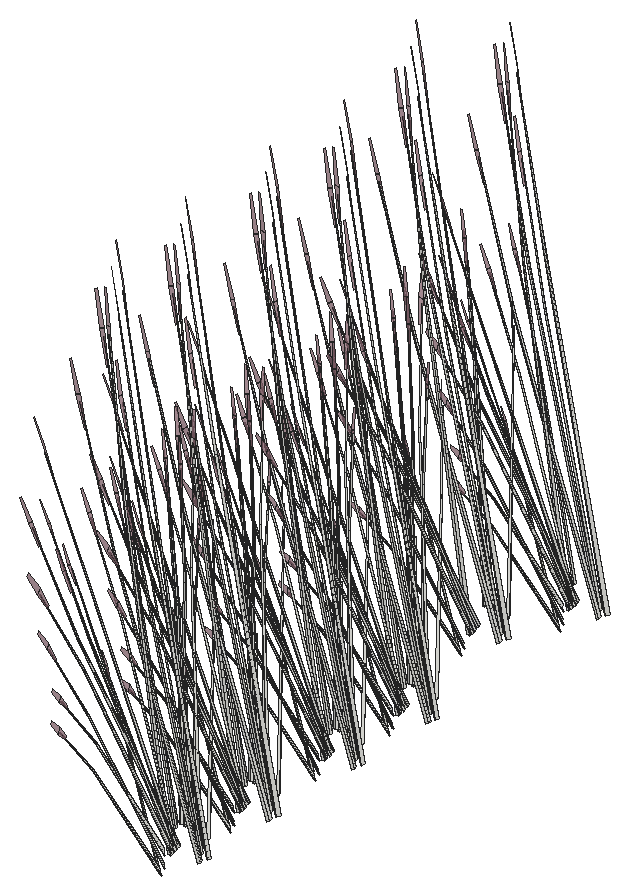
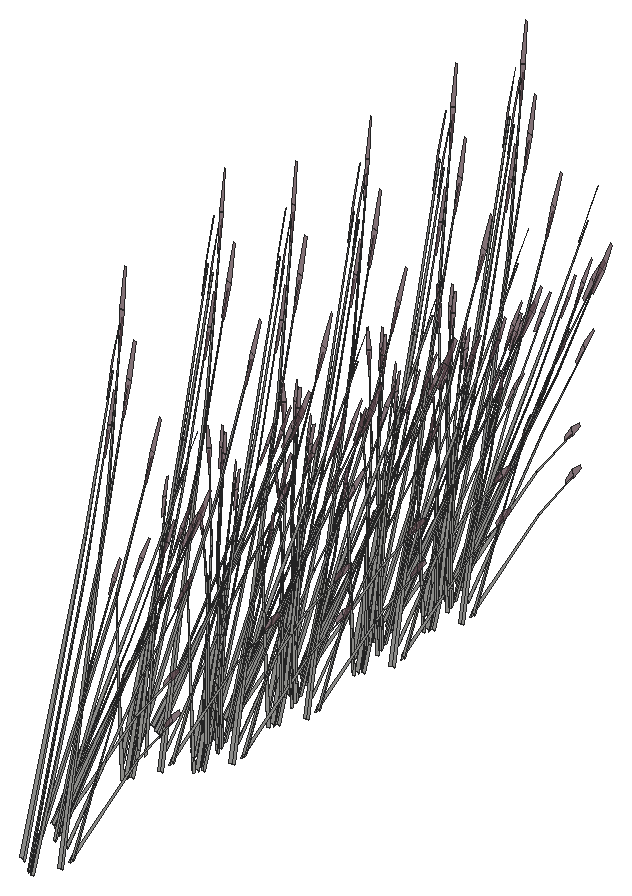
# SketchUp Ruby script. Lengths in inches.
U = 1.inch
M = Sketchup.active_model
def pt(a) = Geom::Point3d.new(a.map { |v| v * U })
def face(e, loops, mat)
  f = e.add_face(loops[0].map { |a| pt(a) })
  loops[1..].each { |l| e.add_face(l.map { |a| pt(a) }).erase! }
  f.material = f.back_material = mat if mat
  f
end
# faces: each face lists its corners as indices into pts; further lists are holes
def faces(e, pts, list, mat = nil) = list.each { |f| face(e, (f[0].is_a?(Array) ? f : [f]).map { |l| l.map { |i| pts[i] } }, mat) }
# xy, xz, yz: faces in a plane at the given z, y or x. An outline is a flat list of corners, or four numbers for a rectangle; further outlines are holes
def ring(l) = l.size == 4 ? [[l[0], l[1]], [l[2], l[1]], [l[2], l[3]], [l[0], l[3]]] : l.each_slice(2).to_a
def flat(e, list, mat, &to3) = list.each { |f| face(e, (f[0].is_a?(Array) ? f : [f]).map { |l| ring(l).map { |u, v| to3.(u, v) } }, mat) }
def xy(e, z, list, mat = nil) = flat(e, list, mat) { |x, y| [x, y, z] }
def xz(e, y, list, mat = nil) = flat(e, list, mat) { |x, z| [x, y, z] }
def yz(e, x, list, mat = nil) = flat(e, list, mat) { |y, z| [x, y, z] }
def lines(e, pts, list) = list.each { |a, b| e.add_line(pt(pts[a]), pt(pts[b])) }
# prism: a flat outline (further loops are holes) pulled along v
def prism(e, loops, v, mat = nil)
  f = face(e, loops, mat); d = Geom::Vector3d.new(v.map { |x| x * U })
  f.pushpull(f.normal.samedirection?(d) ? d.length : -d.length)
end
def box(e, o, s, mat = nil) = prism(e, [[o, [o[0] + s[0], o[1], o[2]], [o[0] + s[0], o[1] + s[1], o[2]], [o[0], o[1] + s[1], o[2]]]], [0, 0, s[2]], mat)
def at(x, y, z, deg = 0) = Geom::Transformation.translation(pt([x, y, z])) * Geom::Transformation.rotation(ORIGIN, Z_AXIS, deg.degrees)
def axes(o, x, y, z) = Geom::Transformation.new([*x, 0, *y, 0, *z, 0, *pt(o).to_a, 1])
def part(name) = M.definitions.add(name)
# library, detail: a bought-in or finely detailed component or shape, given as its bounding box
def library(name, o, s) = part(name).tap { |d| box(d.entities, o, s) }
def detail(e, o, s) = box(e.add_group.entities, o, s)
def put(e, d, t, mat = nil) = e.add_instance(d, t).tap { |i| i.material = mat if mat }
def group(e, t, mat = nil) = e.add_group.tap { |g| g.transformation = t; g.material = mat if mat }.entities
root = M.entities
M.materials.add("LightPink_Translucent").color = [144, 107, 117]
M.materials["LightPink_Translucent"].alpha = 0.75
c1 = part("blade")
p = [[2.15,0.21,22],[0,0.17,0],[0.09,0.45,0],[2.18,0.31,22],[2.29,0.31,22],[0.38,0.45,0],
  [2.48,0.24,33],[2.49,0.24,33],[2.48,0.22,33]]
faces(c1.entities,p,[[0,1,2,3],[4,5,2,3],[6,3,4,7],[8,0,3,6]])
c2 = part("seeds")
p = [[0.3,-0.1,1.38],[-0.01,-0.03,1.59],[-0.01,-0.03,0.03],[0.14,-0.07,-0.07],[0.29,-0.03,3],[0.15,0.01,3.11]]
faces(c2.entities,p,[[0,1,2,3],[1,0,4,5]],"LightPink_Translucent")
c3 = part("blade with seeds")
put(c3.entities,c1,at(0,0,0))
put(c3.entities,c2,axes([2.4,0.25,30.99],[1.5799,-0.05474,1.17369],[-0.12525,1.92788,0.29478],[-0.07173,-0.02425,1.56792]))
put(root,c3,axes([342.42,59.125,6.17],[0.2045,0.20949,1.71376],[-0.94495,0.17636,0.13857],[-0.21357,-0.32887,0.73262]))
put(root,c3,axes([342.16,58.57,4.88],[-0.05417,0.21344,1.43002],[-0.79196,0.17867,-0.30754],[-0.18512,-0.27588,0.61141]))
put(root,c3,axes([343.05,57.4375,7],[-0.01669,0.07821,1.77383],[-0.82314,0.28383,-0.16761],[-0.24223,-0.14508,0.31391]))
put(root,c3,axes([343.02,59.43,7.27],[-0.76283,-0.31537,-0.71045],[0.54213,-0.55263,0.08574],[-0.27638,-0.1883,1.00501]))
put(root,c3,axes([342.75,59.01,6.82],[-0.13817,-0.52554,-0.35414],[0.78985,-0.13877,0.4572],[-0.21215,-0.1506,0.87481]))
put(root,c3,axes([341.52,58.91,3.79],[-0.08666,0.08595,1.76342],[-0.87574,0.18531,-0.26939],[-0.21156,-0.16858,0.30037]))
put(root,c3,axes([342.66,59.45,6.97],[-0.88277,0.1551,-0.51099],[-0.15442,-0.58737,-0.3958],[-0.23711,-0.16832,0.97773]))
put(root,c3,axes([343.28,58.92,7.72],[-0.59706,0.6255,-0.13619],[-0.86465,-0.36036,-0.75594],[-0.30056,-0.17672,1.14864]))
put(root,c3,axes([341.19,59.78,7.02],[0.04505,-0.49615,0.0643],[0.68022,0.0136,0.50621],[-0.26056,-0.05192,0.77189]))
put(root,c3,axes([340.98,59.24,4.42],[-0.25807,0.53277,-0.03893],[-0.79428,-0.16389,-0.17649],[-0.1206,-0.08714,0.58215]))
put(root,c3,axes([340.55,61.68,4.67],[-1.11865,0,0],[0,-0.72922,-0.51607],[0,-0.16609,1.63711]))
put(root,c3,axes([341.65,60.15,7.34],[0.50902,0.40851,0.35414],[-0.58122,0.38671,-0.4572],[-0.29531,-0.05884,0.87481]))
put(root,c3,axes([343.11,62.52,4.35],[-0.9306,-0.10697,-0.62353],[0.19638,-0.65984,-0.16365],[-0.27771,-0.07995,1.37633]))
put(root,c3,axes([342.12,63.53,4.32],[-0.21015,-0.56852,-0.30978],[0.83462,-0.16144,0.30978],[-0.16826,-0.06556,1.38974]))
put(root,c3,axes([341.89,63.77,4.3125],[-0.83726,-0.32623,-0.49651],[0.50045,-0.58498,0],[-0.19069,-0.0743,1.57504]))
put(root,c3,axes([344.17,62.62,4.96],[-0.90324,0.43318,-0.29095],[-0.60064,-0.61207,-0.50002],[-0.22285,-0.06216,1.59708]))
put(root,c3,axes([340.81,61.3,7.34],[0.74348,0.18202,0.35414],[-0.21685,0.53102,-0.4572],[-0.29933,0.04869,0.87481]))
put(root,c3,axes([342.42,68.95,6.17],[0.2045,0.20949,1.71376],[-0.94495,0.17636,0.13857],[-0.21357,-0.32887,0.73262]))
put(root,c3,axes([342.4,64.17,4.67],[-0.55932,0.6538,0],[-0.93577,-0.36461,-0.51607],[-0.21313,-0.08304,1.63711]))
put(root,c3,axes([342.16,68.4,4.88],[-0.05417,0.21344,1.43002],[-0.79196,0.17867,-0.30754],[-0.18512,-0.27588,0.61141]))
put(root,c3,axes([340.23,62.66,7.02],[-0.61415,-0.2744,0.0643],[0.35756,-0.39076,0.50621],[-0.1969,0.12633,0.77189]))
put(root,c3,axes([343.05,67.26,7],[-0.01669,0.07821,1.77383],[-0.82314,0.28383,-0.16761],[-0.24223,-0.14508,0.31391]))
put(root,c3,axes([340.93,62.57,7.34],[0.77872,-0.09325,0.35414],[0.20563,0.53305,-0.4572],[-0.22316,0.14318,0.87481]))
put(root,c3,axes([343.02,69.26,7.27],[-0.76283,-0.31537,-0.71045],[0.54213,-0.55263,0.08574],[-0.27638,-0.1883,1.00501]))
put(root,c3,axes([342.75,68.84,6.82],[-0.13817,-0.52554,-0.35414],[0.78985,-0.13877,0.4572],[-0.21215,-0.1506,0.87481]))
put(root,c3,axes([341.52,68.74,3.79],[-0.08666,0.08595,1.76342],[-0.87574,0.18531,-0.26939],[-0.21156,-0.16858,0.30037]))
put(root,c3,axes([339.17,64.09,7.9375],[0.78943,0.17416,-0.06488],[-0.24284,0.53604,-0.29416],[-0.12912,0.08139,0.97024]))
put(root,c3,axes([342.66,69.27,6.97],[-0.88277,0.1551,-0.51099],[-0.15442,-0.58737,-0.3958],[-0.23711,-0.16832,0.97773]))
put(root,c3,axes([343.28,68.75,7.72],[-0.59706,0.6255,-0.13619],[-0.86465,-0.36036,-0.75594],[-0.30056,-0.17672,1.14864]))
put(root,c3,axes([340.53,62.52,7.33],[0.82753,0.35977,-0.1216],[-0.47675,0.52101,-0.67495],[-0.2338,0.18111,1.02557]))
put(root,c3,axes([340.94,62.95,6.97],[0.22982,0.59576,-0.51099],[-0.87033,0.10422,-0.3958],[-0.24941,0.16002,0.97773]))
put(root,c3,axes([341.4375,63.95,7.02],[-0.73517,-0.0304,0.0643],[0.02016,-0.45906,0.50621],[-0.07693,0.17585,0.77189]))
put(root,c3,axes([341.67,63.99,7.03],[-0.63704,-0.44518,0.48003],[0.67652,-0.38394,0.3958],[-0.11751,0.20886,0.9933]))
put(root,c3,axes([341.48,62.86,6.17],[0.16657,-0.22426,1.71376],[0.69879,0.4641,0.13857],[-0.31524,0.28926,0.73262]))
put(root,c3,axes([341.19,69.61,7.02],[0.04505,-0.49615,0.0643],[0.68022,0.0136,0.50621],[-0.26056,-0.05192,0.77189]))
put(root,c3,axes([339.58,64.02,7.01],[-0.02224,0.12912,1.74944],[0.63107,0.44917,-0.27667],[-0.16521,0.21241,0.14031]))
put(root,c3,axes([340.98,69.07,4.42],[-0.25807,0.53277,-0.03893],[-0.79428,-0.16389,-0.17649],[-0.1206,-0.08714,0.58215]))
put(root,c3,axes([340.55,71.5,4.67],[-1.11865,0,0],[0,-0.72922,-0.51607],[0,-0.16609,1.63711]))
put(root,c3,axes([341.65,69.98,7.34],[0.50902,0.40851,0.35414],[-0.58122,0.38671,-0.4572],[-0.29531,-0.05884,0.87481]))
put(root,c3,axes([341.38,65.11,4.88],[0.28231,-0.10293,1.43002],[0.69701,0.31035,-0.30754],[-0.20746,0.26854,0.61141]))
put(root,c3,axes([343.11,72.35,4.35],[-0.9306,-0.10697,-0.62353],[0.19638,-0.65984,-0.16365],[-0.27771,-0.07995,1.37633]))
put(root,c3,axes([342.12,73.35,4.32],[-0.21015,-0.56852,-0.30978],[0.83462,-0.16144,0.30978],[-0.16826,-0.06556,1.38974]))
put(root,c3,axes([341.89,73.6,4.3125],[-0.83726,-0.32623,-0.49651],[0.50045,-0.58498,0],[-0.19069,-0.0743,1.57504]))
put(root,c3,axes([344.17,72.45,4.96],[-0.90324,0.43318,-0.29095],[-0.60064,-0.61207,-0.50002],[-0.22285,-0.06216,1.59708]))
put(root,c3,axes([340.81,71.125,7.34],[0.74348,0.18202,0.35414],[-0.21685,0.53102,-0.4572],[-0.29933,0.04869,0.87481]))
put(root,c3,axes([342.4,73.99,4.67],[-0.55932,0.6538,0],[-0.93577,-0.36461,-0.51607],[-0.21313,-0.08304,1.63711]))
put(root,c3,axes([340.23,72.48,7.02],[-0.61415,-0.2744,0.0643],[0.35756,-0.39076,0.50621],[-0.1969,0.12633,0.77189]))
put(root,c3,axes([340.93,72.4,7.34],[0.77872,-0.09325,0.35414],[0.20563,0.53305,-0.4572],[-0.22316,0.14318,0.87481]))
put(root,c3,axes([342.42,80.95,6.17],[0.2045,0.20949,1.71376],[-0.94495,0.17636,0.13857],[-0.21357,-0.32887,0.73262]))
put(root,c3,axes([342.16,80.4,4.88],[-0.05417,0.21344,1.43002],[-0.79196,0.17867,-0.30754],[-0.18512,-0.27588,0.61141]))
put(root,c3,axes([339.17,73.91,7.9375],[0.78943,0.17416,-0.06488],[-0.24284,0.53604,-0.29416],[-0.12912,0.08139,0.97024]))
put(root,c3,axes([340.53,72.35,7.33],[0.82753,0.35977,-0.1216],[-0.47675,0.52101,-0.67495],[-0.2338,0.18111,1.02557]))
put(root,c3,axes([340.94,72.78,6.97],[0.22982,0.59576,-0.51099],[-0.87033,0.10422,-0.3958],[-0.24941,0.16002,0.97773]))
put(root,c3,axes([343.05,79.26,7],[-0.01669,0.07821,1.77383],[-0.82314,0.28383,-0.16761],[-0.24223,-0.14508,0.31391]))
put(root,c3,axes([341.4375,73.77,7.02],[-0.73517,-0.0304,0.0643],[0.02016,-0.45906,0.50621],[-0.07693,0.17585,0.77189]))
put(root,c3,axes([341.67,73.81,7.03],[-0.63704,-0.44518,0.48003],[0.67652,-0.38394,0.3958],[-0.11751,0.20886,0.9933]))
put(root,c3,axes([343.02,81.26,7.27],[-0.76283,-0.31537,-0.71045],[0.54213,-0.55263,0.08574],[-0.27638,-0.1883,1.00501]))
put(root,c3,axes([342.75,80.84,6.82],[-0.13817,-0.52554,-0.35414],[0.78985,-0.13877,0.4572],[-0.21215,-0.1506,0.87481]))
put(root,c3,axes([341.48,72.68,6.17],[0.16657,-0.22426,1.71376],[0.69879,0.4641,0.13857],[-0.31524,0.28926,0.73262]))
put(root,c3,axes([341.52,80.74,3.79],[-0.08666,0.08595,1.76342],[-0.87574,0.18531,-0.26939],[-0.21156,-0.16858,0.30037]))
put(root,c3,axes([339.58,73.85,7.01],[-0.02224,0.12912,1.74944],[0.63107,0.44917,-0.27667],[-0.16521,0.21241,0.14031]))
put(root,c3,axes([342.66,81.27,6.97],[-0.88277,0.1551,-0.51099],[-0.15442,-0.58737,-0.3958],[-0.23711,-0.16832,0.97773]))
put(root,c3,axes([343.28,80.75,7.72],[-0.59706,0.6255,-0.13619],[-0.86465,-0.36036,-0.75594],[-0.30056,-0.17672,1.14864]))
put(root,c3,axes([341.38,74.9375,4.88],[0.28231,-0.10293,1.43002],[0.69701,0.31035,-0.30754],[-0.20746,0.26854,0.61141]))
put(root,c3,axes([341.19,81.61,7.02],[0.04505,-0.49615,0.0643],[0.68022,0.0136,0.50621],[-0.26056,-0.05192,0.77189]))
put(root,c3,axes([340.98,81.07,4.42],[-0.25807,0.53277,-0.03893],[-0.79428,-0.16389,-0.17649],[-0.1206,-0.08714,0.58215]))
put(root,c3,axes([340.55,83.5,4.67],[-1.11865,0,0],[0,-0.72922,-0.51607],[0,-0.16609,1.63711]))
put(root,c3,axes([341.65,81.98,7.34],[0.50902,0.40851,0.35414],[-0.58122,0.38671,-0.4572],[-0.29531,-0.05884,0.87481]))
put(root,c3,axes([343.11,84.35,4.35],[-0.9306,-0.10697,-0.62353],[0.19638,-0.65984,-0.16365],[-0.27771,-0.07995,1.37633]))
put(root,c3,axes([342.12,85.35,4.32],[-0.21015,-0.56852,-0.30978],[0.83462,-0.16144,0.30978],[-0.16826,-0.06556,1.38974]))
put(root,c3,axes([341.89,85.6,4.3125],[-0.83726,-0.32623,-0.49651],[0.50045,-0.58498,0],[-0.19069,-0.0743,1.57504]))
put(root,c3,axes([344.17,84.45,4.96],[-0.90324,0.43318,-0.29095],[-0.60064,-0.61207,-0.50002],[-0.22285,-0.06216,1.59708]))
put(root,c3,axes([340.81,83.125,7.34],[0.74348,0.18202,0.35414],[-0.21685,0.53102,-0.4572],[-0.29933,0.04869,0.87481]))
put(root,c3,axes([342.4,85.99,4.67],[-0.55932,0.6538,0],[-0.93577,-0.36461,-0.51607],[-0.21313,-0.08304,1.63711]))
put(root,c3,axes([342.42,91.42,6.17],[0.2045,0.20949,1.71376],[-0.94495,0.17636,0.13857],[-0.21357,-0.32887,0.73262]))
put(root,c3,axes([342.16,90.87,4.88],[-0.05417,0.21344,1.43002],[-0.79196,0.17867,-0.30754],[-0.18512,-0.27588,0.61141]))
put(root,c3,axes([340.23,84.48,7.02],[-0.61415,-0.2744,0.0643],[0.35756,-0.39076,0.50621],[-0.1969,0.12633,0.77189]))
put(root,c3,axes([340.93,84.4,7.34],[0.77872,-0.09325,0.35414],[0.20563,0.53305,-0.4572],[-0.22316,0.14318,0.87481]))
put(root,c3,axes([343.05,89.73,7],[-0.01669,0.07821,1.77383],[-0.82314,0.28383,-0.16761],[-0.24223,-0.14508,0.31391]))
put(root,c3,axes([339.17,85.91,7.9375],[0.78943,0.17416,-0.06488],[-0.24284,0.53604,-0.29416],[-0.12912,0.08139,0.97024]))
put(root,c3,axes([343.02,91.73,7.27],[-0.76283,-0.31537,-0.71045],[0.54213,-0.55263,0.08574],[-0.27638,-0.1883,1.00501]))
put(root,c3,axes([342.75,91.3125,6.82],[-0.13817,-0.52554,-0.35414],[0.78985,-0.13877,0.4572],[-0.21215,-0.1506,0.87481]))
put(root,c3,axes([340.53,84.35,7.33],[0.82753,0.35977,-0.1216],[-0.47675,0.52101,-0.67495],[-0.2338,0.18111,1.02557]))
put(root,c3,axes([341.52,91.21,3.79],[-0.08666,0.08595,1.76342],[-0.87574,0.18531,-0.26939],[-0.21156,-0.16858,0.30037]))
put(root,c3,axes([340.94,84.78,6.97],[0.22982,0.59576,-0.51099],[-0.87033,0.10422,-0.3958],[-0.24941,0.16002,0.97773]))
put(root,c3,axes([342.66,91.75,6.97],[-0.88277,0.1551,-0.51099],[-0.15442,-0.58737,-0.3958],[-0.23711,-0.16832,0.97773]))
put(root,c3,axes([341.4375,85.77,7.02],[-0.73517,-0.0304,0.0643],[0.02016,-0.45906,0.50621],[-0.07693,0.17585,0.77189]))
put(root,c3,axes([343.28,91.22,7.72],[-0.59706,0.6255,-0.13619],[-0.86465,-0.36036,-0.75594],[-0.30056,-0.17672,1.14864]))
put(root,c3,axes([341.67,85.81,7.03],[-0.63704,-0.44518,0.48003],[0.67652,-0.38394,0.3958],[-0.11751,0.20886,0.9933]))
put(root,c3,axes([341.48,84.68,6.17],[0.16657,-0.22426,1.71376],[0.69879,0.4641,0.13857],[-0.31524,0.28926,0.73262]))
put(root,c3,axes([339.58,85.85,7.01],[-0.02224,0.12912,1.74944],[0.63107,0.44917,-0.27667],[-0.16521,0.21241,0.14031]))
put(root,c3,axes([341.19,92.08,7.02],[0.04505,-0.49615,0.0643],[0.68022,0.0136,0.50621],[-0.26056,-0.05192,0.77189]))
put(root,c3,axes([340.98,91.54,4.42],[-0.25807,0.53277,-0.03893],[-0.79428,-0.16389,-0.17649],[-0.1206,-0.08714,0.58215]))
put(root,c3,axes([340.55,93.97,4.67],[-1.11865,0,0],[0,-0.72922,-0.51607],[0,-0.16609,1.63711]))
put(root,c3,axes([341.38,86.9375,4.88],[0.28231,-0.10293,1.43002],[0.69701,0.31035,-0.30754],[-0.20746,0.26854,0.61141]))
put(root,c3,axes([341.65,92.45,7.34],[0.50902,0.40851,0.35414],[-0.58122,0.38671,-0.4572],[-0.29531,-0.05884,0.87481]))
put(root,c3,axes([343.11,94.82,4.35],[-0.9306,-0.10697,-0.62353],[0.19638,-0.65984,-0.16365],[-0.27771,-0.07995,1.37633]))
put(root,c3,axes([342.12,95.83,4.32],[-0.21015,-0.56852,-0.30978],[0.83462,-0.16144,0.30978],[-0.16826,-0.06556,1.38974]))
put(root,c3,axes([341.89,96.07,4.3125],[-0.83726,-0.32623,-0.49651],[0.50045,-0.58498,0],[-0.19069,-0.0743,1.57504]))
put(root,c3,axes([344.17,94.92,4.96],[-0.90324,0.43318,-0.29095],[-0.60064,-0.61207,-0.50002],[-0.22285,-0.06216,1.59708]))
put(root,c3,axes([340.81,93.6,7.34],[0.74348,0.18202,0.35414],[-0.21685,0.53102,-0.4572],[-0.29933,0.04869,0.87481]))
put(root,c3,axes([342.4,96.46,4.67],[-0.55932,0.6538,0],[-0.93577,-0.36461,-0.51607],[-0.21313,-0.08304,1.63711]))
put(root,c3,axes([342.42,101.49,9.875],[0.2045,0.20949,1.71376],[-0.94495,0.17636,0.13857],[-0.21357,-0.32887,0.73262]))
put(root,c3,axes([342.16,100.9375,8.59],[-0.05417,0.21344,1.43002],[-0.79196,0.17867,-0.30754],[-0.18512,-0.27588,0.61141]))
put(root,c3,axes([340.23,94.95,7.02],[-0.61415,-0.2744,0.0643],[0.35756,-0.39076,0.50621],[-0.1969,0.12633,0.77189]))
put(root,c3,axes([340.93,94.87,7.34],[0.77872,-0.09325,0.35414],[0.20563,0.53305,-0.4572],[-0.22316,0.14318,0.87481]))
put(root,c3,axes([343.02,101.8,10.98],[-0.76283,-0.31537,-0.71045],[0.54213,-0.55263,0.08574],[-0.27638,-0.1883,1.00501]))
put(root,c3,axes([342.75,101.38,10.53],[-0.13817,-0.52554,-0.35414],[0.78985,-0.13877,0.4572],[-0.21215,-0.1506,0.87481]))
put(root,c3,axes([339.17,96.38,7.9375],[0.78943,0.17416,-0.06488],[-0.24284,0.53604,-0.29416],[-0.12912,0.08139,0.97024]))
put(root,c3,axes([341.52,101.28,7.49],[-0.08666,0.08595,1.76342],[-0.87574,0.18531,-0.26939],[-0.21156,-0.16858,0.30037]))
put(root,c3,axes([340.53,94.82,7.33],[0.82753,0.35977,-0.1216],[-0.47675,0.52101,-0.67495],[-0.2338,0.18111,1.02557]))
put(root,c3,axes([342.66,101.8125,10.68],[-0.88277,0.1551,-0.51099],[-0.15442,-0.58737,-0.3958],[-0.23711,-0.16832,0.97773]))
put(root,c3,axes([340.94,95.25,6.97],[0.22982,0.59576,-0.51099],[-0.87033,0.10422,-0.3958],[-0.24941,0.16002,0.97773]))
put(root,c3,axes([341.4375,96.24,7.02],[-0.73517,-0.0304,0.0643],[0.02016,-0.45906,0.50621],[-0.07693,0.17585,0.77189]))
put(root,c3,axes([341.67,96.29,7.03],[-0.63704,-0.44518,0.48003],[0.67652,-0.38394,0.3958],[-0.11751,0.20886,0.9933]))
put(root,c3,axes([341.48,95.16,6.17],[0.16657,-0.22426,1.71376],[0.69879,0.4641,0.13857],[-0.31524,0.28926,0.73262]))
put(root,c3,axes([339.58,96.32,7.01],[-0.02224,0.12912,1.74944],[0.63107,0.44917,-0.27667],[-0.16521,0.21241,0.14031]))
put(root,c3,axes([340.98,101.61,8.13],[-0.25807,0.53277,-0.03893],[-0.79428,-0.16389,-0.17649],[-0.1206,-0.08714,0.58215]))
put(root,c3,axes([340.55,104.04,8.375],[-1.11865,0,0],[0,-0.72922,-0.51607],[0,-0.16609,1.63711]))
put(root,c3,axes([341.38,97.41,4.88],[0.28231,-0.10293,1.43002],[0.69701,0.31035,-0.30754],[-0.20746,0.26854,0.61141]))
put(root,c3,axes([343.11,104.89,8.06],[-0.9306,-0.10697,-0.62353],[0.19638,-0.65984,-0.16365],[-0.27771,-0.07995,1.37633]))
put(root,c3,axes([342.12,105.89,8.03],[-0.21015,-0.56852,-0.30978],[0.83462,-0.16144,0.30978],[-0.16826,-0.06556,1.38974]))
put(root,c3,axes([341.89,106.14,8.02],[-0.83726,-0.32623,-0.49651],[0.50045,-0.58498,0],[-0.19069,-0.0743,1.57504]))
put(root,c3,axes([344.17,104.99,8.67],[-0.90324,0.43318,-0.29095],[-0.60064,-0.61207,-0.50002],[-0.22285,-0.06216,1.59708]))
put(root,c3,axes([342.4,106.53,8.375],[-0.55932,0.6538,0],[-0.93577,-0.36461,-0.51607],[-0.21313,-0.08304,1.63711]))
put(root,c3,axes([340.94,105.32,10.68],[0.22982,0.59576,-0.51099],[-0.87033,0.10422,-0.3958],[-0.24941,0.16002,0.97773]))
put(root,c3,axes([342.42,115.5,6.17],[0.2045,0.20949,1.71376],[-0.94495,0.17636,0.13857],[-0.21357,-0.32887,0.73262]))
put(root,c3,axes([341.48,105.22,9.875],[0.16657,-0.22426,1.71376],[0.69879,0.4641,0.13857],[-0.31524,0.28926,0.73262]))
put(root,c3,axes([342.16,114.94,4.88],[-0.05417,0.21344,1.43002],[-0.79196,0.17867,-0.30754],[-0.18512,-0.27588,0.61141]))
put(root,c3,axes([343.05,113.81,7],[-0.01669,0.07821,1.77383],[-0.82314,0.28383,-0.16761],[-0.24223,-0.14508,0.31391]))
put(root,c3,axes([343.02,115.8,7.27],[-0.76283,-0.31537,-0.71045],[0.54213,-0.55263,0.08574],[-0.27638,-0.1883,1.00501]))
put(root,c3,axes([342.75,115.39,6.82],[-0.13817,-0.52554,-0.35414],[0.78985,-0.13877,0.4572],[-0.21215,-0.1506,0.87481]))
put(root,c3,axes([341.38,107.48,8.59],[0.28231,-0.10293,1.43002],[0.69701,0.31035,-0.30754],[-0.20746,0.26854,0.61141]))
put(root,c3,axes([341.52,115.29,3.79],[-0.08666,0.08595,1.76342],[-0.87574,0.18531,-0.26939],[-0.21156,-0.16858,0.30037]))
put(root,c3,axes([342.66,115.82,6.97],[-0.88277,0.1551,-0.51099],[-0.15442,-0.58737,-0.3958],[-0.23711,-0.16832,0.97773]))
put(root,c3,axes([343.28,115.3,7.72],[-0.59706,0.6255,-0.13619],[-0.86465,-0.36036,-0.75594],[-0.30056,-0.17672,1.14864]))
put(root,c3,axes([341.19,116.16,7.02],[0.04505,-0.49615,0.0643],[0.68022,0.0136,0.50621],[-0.26056,-0.05192,0.77189]))
put(root,c3,axes([340.98,115.62,4.42],[-0.25807,0.53277,-0.03893],[-0.79428,-0.16389,-0.17649],[-0.1206,-0.08714,0.58215]))
put(root,c3,axes([340.55,118.05,4.67],[-1.11865,0,0],[0,-0.72922,-0.51607],[0,-0.16609,1.63711]))
put(root,c3,axes([341.65,116.53,7.34],[0.50902,0.40851,0.35414],[-0.58122,0.38671,-0.4572],[-0.29531,-0.05884,0.87481]))
put(root,c3,axes([343.11,118.9,4.35],[-0.9306,-0.10697,-0.62353],[0.19638,-0.65984,-0.16365],[-0.27771,-0.07995,1.37633]))
put(root,c3,axes([342.12,119.9,4.32],[-0.21015,-0.56852,-0.30978],[0.83462,-0.16144,0.30978],[-0.16826,-0.06556,1.38974]))
put(root,c3,axes([341.89,120.14,4.3125],[-0.83726,-0.32623,-0.49651],[0.50045,-0.58498,0],[-0.19069,-0.0743,1.57504]))
put(root,c3,axes([344.17,118.99,4.96],[-0.90324,0.43318,-0.29095],[-0.60064,-0.61207,-0.50002],[-0.22285,-0.06216,1.59708]))
put(root,c3,axes([340.81,117.67,7.34],[0.74348,0.18202,0.35414],[-0.21685,0.53102,-0.4572],[-0.29933,0.04869,0.87481]))
